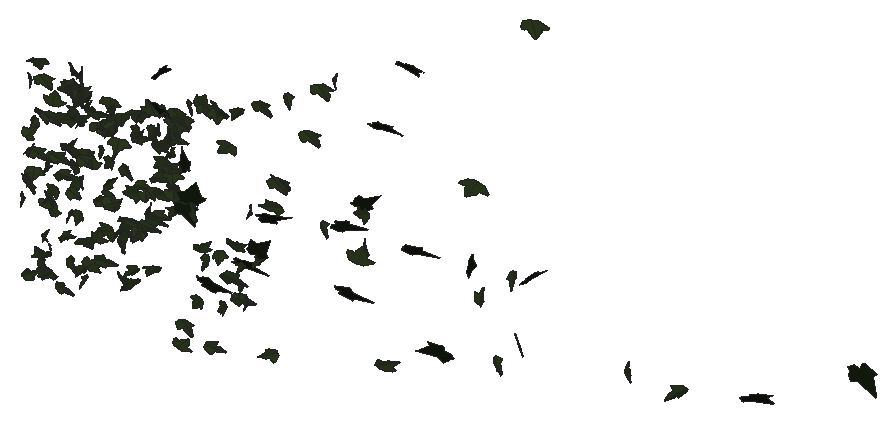
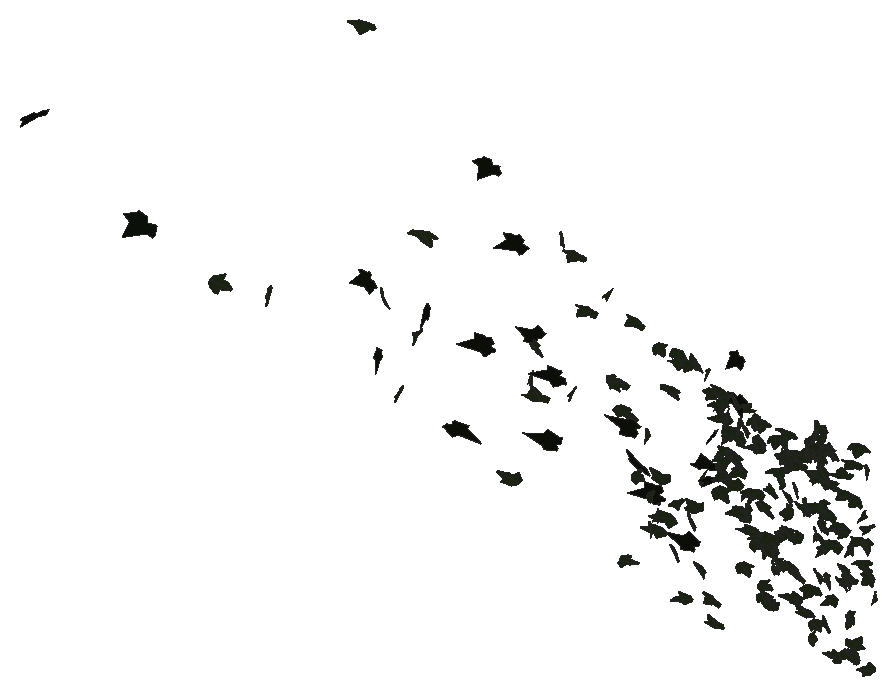
# SketchUp Ruby script. Lengths in millimetres.
U = 1.mm
M = Sketchup.active_model
def pt(a) = Geom::Point3d.new(a.map { |v| v * U })
def face(e, loops, mat)
  f = e.add_face(loops[0].map { |a| pt(a) })
  loops[1..].each { |l| e.add_face(l.map { |a| pt(a) }).erase! }
  f.material = f.back_material = mat if mat
  f
end
# faces: each face lists its corners as indices into pts; further lists are holes
def faces(e, pts, list, mat = nil) = list.each { |f| face(e, (f[0].is_a?(Array) ? f : [f]).map { |l| l.map { |i| pts[i] } }, mat) }
# xy, xz, yz: faces in a plane at the given z, y or x. An outline is a flat list of corners, or four numbers for a rectangle; further outlines are holes
def ring(l) = l.size == 4 ? [[l[0], l[1]], [l[2], l[1]], [l[2], l[3]], [l[0], l[3]]] : l.each_slice(2).to_a
def flat(e, list, mat, &to3) = list.each { |f| face(e, (f[0].is_a?(Array) ? f : [f]).map { |l| ring(l).map { |u, v| to3.(u, v) } }, mat) }
def xy(e, z, list, mat = nil) = flat(e, list, mat) { |x, y| [x, y, z] }
def xz(e, y, list, mat = nil) = flat(e, list, mat) { |x, z| [x, y, z] }
def yz(e, x, list, mat = nil) = flat(e, list, mat) { |y, z| [x, y, z] }
def lines(e, pts, list) = list.each { |a, b| e.add_line(pt(pts[a]), pt(pts[b])) }
# prism: a flat outline (further loops are holes) pulled along v
def prism(e, loops, v, mat = nil)
  f = face(e, loops, mat); d = Geom::Vector3d.new(v.map { |x| x * U })
  f.pushpull(f.normal.samedirection?(d) ? d.length : -d.length)
end
def box(e, o, s, mat = nil) = prism(e, [[o, [o[0] + s[0], o[1], o[2]], [o[0] + s[0], o[1] + s[1], o[2]], [o[0], o[1] + s[1], o[2]]]], [0, 0, s[2]], mat)
def at(x, y, z, deg = 0) = Geom::Transformation.translation(pt([x, y, z])) * Geom::Transformation.rotation(ORIGIN, Z_AXIS, deg.degrees)
def axes(o, x, y, z) = Geom::Transformation.new([*x, 0, *y, 0, *z, 0, *pt(o).to_a, 1])
def part(name) = M.definitions.add(name)
# library, detail: a bought-in or finely detailed component or shape, given as its bounding box
def library(name, o, s) = part(name).tap { |d| box(d.entities, o, s) }
def detail(e, o, s) = box(e.add_group.entities, o, s)
def put(e, d, t, mat = nil) = e.add_instance(d, t).tap { |i| i.material = mat if mat }
def group(e, t, mat = nil) = e.add_group.tap { |g| g.transformation = t; g.material = mat if mat }.entities
root = M.entities
M.materials.add("efeu1").color = [18, 25, 13]
M.materials.add("efeu2").color = [43, 57, 29]
c1 = part("ivyleaf_10")
p = [[0,12.8,-0.8],[-1.5,51.3,-10.9],[-4.9,51,-11.6],[-13.6,26.5,-7.3],[-13.2,15.9,-4.6],[-21.1,19.3,-7.2],
  [-29.5,16.3,-8.3],[-29.2,8.3,-6.2],[-19.7,-9.8,0.5],[-7.6,-13,4],[1,-12.2,5.8],[-0.4,51.1,-11.1],
  [-1.5,51.1,-10.9],[1,-12.4,5.9],[16.9,-12.4,3.5],[35.1,9.1,-5.1],[35,12.9,-6.1],[20.5,16.4,-4.9],
  [15.8,15,-3.8],[15.3,27.6,-7.1],[12.8,31.3,-7.8]]
faces(c1.entities,p,[[0,1,2,3,4,5,6,7,8,9,10],[11,12,0,13,14,15,16,17,18,19,20]],"efeu2")
c2 = part("ivyleaf_9")
p = [[39.1,54.8,31.7],[34.5,51.8,30.2],[-5.3,25.2,17.3],[-17.9,28.3,20.9],[-21.6,21.7,17],[-20.2,4.3,5.3],
  [-22.9,-0.3,2.5],[-17.1,-4,-0.6],[-2,-2.1,-1.2],[-0.7,-15.4,-10.1],[16.6,-22.3,-16.7],[21.1,-15.1,-12.5],
  [32.7,-10.7,-11],[46.1,-1.8,-6.6],[30.8,11.2,3.8]]
faces(c2.entities,p,[[0,1,2,3,4,5,6,7,8,9,10,11,12,13,14]],"efeu1")
put(root,c1,axes([1239.6,1052.6,288.6],[0.16019,-0.32764,-0.55839],[0.05337,0.5644,-0.32694],[1.23101,0.01817,0.08684]))
put(root,c1,axes([1265.3,1054.1,359.1],[0.11388,-0.04414,-0.63331],[-0.61555,0.54526,-0.06856],[1.03969,0.32766,0.02877]))
put(root,c1,axes([1251.3,1065.3,348],[-0.8892,0.39163,-0.24482],[0.3663,-0.15147,-0.6096],[-0.79905,-0.50525,-0.00702]))
put(root,c1,axes([1263.4,1066.4,467.4],[-0.03795,-0.71606,-0.12535],[0.02924,0.12496,-0.71624],[1.38322,-0.02229,0.0117]))
put(root,c1,axes([1252.7,1059.1,25.1],[-0.0891,-0.22264,0.63889],[0.20902,0.62942,0.22739],[-1.27057,0.11916,-0.0074]))
put(root,c1,axes([1256.2,1056.7,514.5],[0.46165,0.21093,-0.58955],[0.47216,0.54812,0.29818],[1.09414,-0.32553,0.12007]))
put(root,c1,axes([1273.6,1051.8,714.6],[0.36307,-0.38358,-0.48797],[-0.15599,0.49046,-0.41758],[1.17093,0.18427,0.09567]))
put(root,c1,axes([1269,1079.3,563],[0.15492,0.36895,-0.52964],[-0.1698,-0.52228,-0.37753],[-1.21667,0.11987,-0.01475]))
put(root,c1,axes([1275.1,1067.1,395.9],[0.8809,0.45478,-0.11108],[-0.15445,-0.0759,-0.64888],[-0.87748,0.46991,0.0027]))
put(root,c1,axes([1301.5,1079.7,102.7],[-0.83149,-0.33084,-0.35437],[-0.54732,-0.20719,0.54798],[-0.74282,0.523,-0.00709]))
put(root,c1,axes([1298.2,1060.5,785.8],[-1.01122,-0.36546,-0.08051],[0.13135,0.04172,-0.64486],[0.70001,-0.53577,0.0047]))
put(root,c1,axes([1280.6,1062.8,464.6],[0.59403,0.32673,0.47763],[0.61749,0.35055,-0.45183],[-0.91197,0.45018,0.00518]))
put(root,c1,axes([1300.4,1067.7,604.8],[-1.04499,0.31547,-0.19176],[0.30709,-0.10406,-0.63318],[-0.63197,-0.57221,0.00942]))
put(root,c1,axes([1297.4,1077.6,87.6],[0.62423,-0.2916,0.48272],[0.70851,-0.30752,-0.43871],[0.80626,0.49601,0.01179]))
put(root,c1,axes([1339.7,1065.9,59.1],[-0.8146,-0.17943,0.4451],[-0.7818,-0.17138,-0.46411],[0.47224,-0.59324,-0.00055]))
put(root,c1,axes([1306.1,1065.6,725.5],[0.86618,0.34796,0.36773],[0.54576,0.23032,-0.57285],[-0.79405,0.53787,0.00741]))
put(root,c1,axes([1325,1068.4,195.5],[0.1336,-0.59789,0.21849],[0.09631,-0.21388,-0.60152],[1.20767,0.0832,0.0238]))
put(root,c1,axes([1323.1,1068,63.3],[1.1405,-0.22119,-0.03341],[-0.05398,0.01964,-0.63871],[0.42231,0.59986,0.00859]))
put(root,c1,axes([1328,1060.2,425.4],[-0.0579,-0.29378,-0.60787],[0.16347,0.60186,-0.29517],[1.27448,-0.09054,0.01024]))
put(root,c1,axes([1335.3,1065,320],[-0.00784,-0.64851,-0.13381],[-0.01464,0.13385,-0.64847],[1.26016,-0.00248,-0.00837]))
put(root,c1,axes([1327.9,1068.9,160.2],[-0.63818,0.13904,0.55531],[0.74319,-0.41503,0.33971],[0.79666,0.49856,0.12793]))
put(root,c1,axes([1355.5,1053.2,316.1],[-0.27159,0.28396,-0.56339],[-0.60895,0.46526,0.31554],[1.03488,0.34829,0.03782]))
put(root,c1,axes([1333.9,1055.8,299.1],[0.71852,0.4355,-0.28324],[0.35775,0.21189,0.57636],[0.92173,-0.42173,-0.00291]))
put(root,c1,axes([1352.4,1069.9,352],[0.85257,-0.40554,-0.30883],[-0.43829,0.20578,-0.60426],[0.86549,0.50369,-0.00178]))
put(root,c1,axes([1332,1064.8,606.9],[0.80832,0.20292,0.45096],[0.74312,0.22718,-0.46996],[-0.57753,0.57632,0.02647]))
put(root,c1,axes([1357.4,1058.1,281],[1.04144,-0.3876,0.19874],[-0.29534,0.12469,0.67047],[-0.7746,-0.56867,0.01156]))
put(root,c1,axes([1356.4,1059.7,661.7],[1.04902,0.35634,-0.13418],[0.20507,0.08045,0.65628],[0.69505,-0.56155,0.00888]))
put(root,c1,axes([1349.1,1057.5,467.3],[0.3398,0.16685,-0.59298],[0.84375,0.39384,0.2443],[0.81397,-0.4779,-0.0057]))
put(root,c1,axes([1364.9,1055.4,480.9],[0.44094,0.27516,0.53506],[0.6765,0.40001,-0.35962],[-0.92391,0.42422,-0.00796]))
put(root,c1,axes([1411.9,1066.6,621],[0.66701,0.02989,-0.56874],[-1.08392,0.01961,-0.34992],[0.00198,0.66776,0.03573]))
put(root,c1,axes([1379.9,1066,418.4],[-0.48841,-0.15825,-0.61335],[1.04911,0.27023,-0.30036],[0.59392,-0.60748,0.02617]))
put(root,c1,axes([1374.9,1064.6,27.8],[0.19939,-0.05457,0.6283],[1.20027,0.00729,-0.10452],[0.00334,0.63693,0.05503]))
put(root,c1,axes([1415.5,1057.8,736.9],[0.50411,-0.35751,-0.46842],[-0.40172,0.42193,-0.44138],[1.04707,0.334,0.05618]))
put(root,c1,axes([1427.7,1059.4,733.6],[0.77838,-0.12558,-0.5347],[-0.95042,0.19254,-0.42719],[0.43522,0.64506,0.02342]))
put(root,c1,axes([1403.3,1052.5,218.6],[-0.32331,-0.2444,-0.60156],[0.58505,0.51743,-0.29703],[1.0885,-0.35071,-0.01903]))
put(root,c1,axes([1401.8,1069.3,518.8],[-0.97641,0.19167,-0.37538],[0.6599,-0.14427,-0.54755],[-0.45606,-0.61911,0.01138]))
put(root,c1,axes([1417.4,1066.8,292.8],[0.34392,-0.66787,0.01791],[0.00895,-0.01728,-0.69189],[1.27152,0.18077,0.00002]))
put(root,c1,axes([1416.8,1057.1,735.4],[-0.68286,0.52593,0.01901],[-0.02016,0.01579,-0.63666],[-1.0014,-0.35895,-0.00015]))
put(root,c1,axes([1416.9,1057.1,743],[-0.0608,-0.32113,-0.5712],[0.49185,0.51935,-0.30643],[1.14604,-0.23993,0.10121]))
put(root,c1,axes([1436.8,1060.3,799.3],[-0.86681,0.33583,0.4292],[-0.67636,0.24103,-0.56572],[-0.78632,-0.57754,0.01348]))
put(root,c1,axes([1429.1,1068.7,546.8],[-0.0112,-0.63791,0.03298],[0.00317,-0.033,-0.63793],[1.21569,-0.00579,0.00197]))
put(root,c1,axes([1444,1059.5,465.6],[0.24965,-0.12149,-0.63926],[-0.66353,0.53749,-0.17369],[1.04565,0.37008,0.04241]))
put(root,c1,axes([1439.1,1061.6,655.6],[0.79728,-0.3409,-0.40351],[-0.50996,0.30669,-0.53728],[0.86641,0.49422,0.05508]))
put(root,c1,axes([1414.1,1069.8,131],[0.54991,-0.24192,0.60536],[0.94435,-0.34786,-0.37585],[0.80472,0.57354,0.02739]))
put(root,c1,axes([1441.6,1064.2,700.2],[-1.03182,0.29658,0.16266],[-0.33597,0.01404,-0.61399],[-0.54914,-0.56585,0.07002]))
put(root,c1,axes([1429.4,1052,381.2],[0.19203,0.49755,0.43375],[0.19197,0.42201,-0.50755],[-1.2415,0.14221,-0.01139]))
put(root,c1,axes([1449.6,1060,418.3],[0.69375,-0.5007,-0.32821],[-0.37923,0.26089,-0.6193],[1.07446,0.41537,-0.00666]))
put(root,c1,axes([1449.6,1063.9,732.7],[-1.18296,-0.1435,0.01032],[-0.02191,0.004,-0.63788],[0.27294,-0.62163,-0.00649]))
put(root,c1,axes([1447.3,1057.2,757.7],[-0.83861,0.45851,0.01765],[-0.04594,0.00127,-0.6357],[-0.87207,-0.44098,0.01652]))
put(root,c1,axes([1444.6,1072.1,298.6],[0.93219,-0.42809,0.11067],[0.16016,-0.07188,-0.65051],[0.82615,0.49698,0.00124]))
put(root,c1,axes([1453.6,1064.8,709.4],[0.25157,-0.58425,-0.21694],[0.01868,0.22369,-0.59645],[1.18598,0.12041,0.05541]))
put(root,c1,axes([1440.5,1067.3,629],[-0.25397,-0.43712,0.49629],[0.55076,0.41665,0.44479],[-1.13178,0.30085,0.10509]))
put(root,c1,axes([1464.4,1070.6,119.1],[-0.29458,-0.51963,0.38028],[-0.07904,-0.38224,-0.53922],[1.22295,-0.14987,0.05675]))
put(root,c1,axes([1472.2,1051.3,420.4],[0.04343,-0.05324,0.7025],[-0.85764,0.53918,0.0555],[-1.03067,-0.45091,-0.01658]))
put(root,c1,axes([1461.3,1058.7,632.7],[-0.09736,-0.50073,-0.41595],[0.16387,0.40837,-0.50219],[1.22802,-0.09419,0.03403]))
put(root,c1,axes([1466.8,1056,771.8],[-0.50304,0.52876,0.26016],[-0.29957,0.21143,-0.58963],[-1.08081,-0.30471,0.04234]))
put(root,c1,axes([1464.7,1058,806.1],[0.14117,-0.5951,-0.25983],[0.07153,0.26502,-0.59624],[1.23377,0.05273,0.0643]))
put(root,c1,axes([1460.2,1084.6,75],[0.15411,-0.34471,0.5667],[0.30524,-0.54379,-0.35369],[1.22494,0.17887,0.01684]))
put(root,c1,axes([1455.1,1062.4,521.9],[-0.7574,-0.23527,-0.49108],[0.82287,0.23322,-0.46211],[0.62998,-0.58748,0.01321]))
put(root,c1,axes([1470.7,1062.7,714.4],[0.48976,-0.56848,-0.14836],[-0.00086,0.16178,-0.62067],[1.11816,0.24912,0.0645]))
put(root,c1,axes([1484.7,1052.8,745.3],[-0.07381,0.49339,0.40523],[-0.19245,0.3961,-0.49196],[-1.19979,-0.09389,0.05398]))
put(root,c1,axes([1474.8,1051.6,509.5],[0.40819,0.53764,0.39935],[0.27462,0.37239,-0.57883],[-1.2447,0.25848,0.00325]))
put(root,c1,axes([1483.2,1057.8,227.8],[-0.91923,-0.41566,-0.28145],[0.40242,0.18578,-0.63722],[0.86649,-0.52724,-0.00264]))
put(root,c1,axes([1490.9,1063.8,702.1],[-0.0473,-0.6374,-0.01661],[-0.00346,0.01669,-0.63788],[1.21351,-0.0248,-0.00246]))
put(root,c1,axes([1495.6,1060.7,732.5],[0.06628,-0.62539,-0.12878],[0.00532,0.12912,-0.62629],[1.21521,0.03354,0.00977]))
put(root,c1,axes([1494.1,1072.2,523.6],[0.57051,-0.49721,0.28868],[0.2419,-0.2602,-0.58014],[1.06716,0.3248,-0.02283]))
put(root,c1,axes([1506.7,1065.1,494.2],[1.02645,-0.14786,0.33847],[-0.62285,0.08644,0.55923],[-0.32593,-0.63085,-0.00271]))
put(root,c1,axes([1488.7,1065.2,140.1],[1.00816,-0.08575,-0.43916],[0.83742,-0.02382,0.53539],[-0.15472,-0.68767,0.03621]))
put(root,c1,axes([1500,1060.9,677.8],[-0.13491,-0.19303,0.65615],[1.15214,0.28929,0.1505],[-0.60579,0.59318,0.14012]))
put(root,c1,axes([1528.3,1058.7,247.3],[1.16473,-0.24836,0.05896],[-0.08475,0.04695,0.65992],[-0.47837,-0.61303,0.02665]))
put(root,c1,axes([1532.2,1052.7,381.8],[0.06111,-0.15718,0.61639],[0.04673,0.61702,0.15606],[-1.20976,0.01589,0.03717]))
put(root,c1,axes([1526.4,1058,641.1],[0.85884,0.33707,0.3113],[0.49371,0.17273,-0.56306],[-0.72028,0.5203,-0.01475]))
put(root,c1,axes([1545.7,1058,560.4],[0.43766,-0.53729,-0.27231],[-0.15774,0.26049,-0.58395],[1.1355,0.24327,0.02384]))
put(root,c1,axes([1564.7,1069.6,286.2],[0.82248,-0.30044,-0.52789],[-0.81753,0.30687,-0.52631],[0.8173,0.60931,0.00478]))
put(root,c1,axes([1532.8,1061.7,174.4],[0.00208,-0.01802,0.64676],[1.0337,0.3515,0.00888],[-0.66918,0.54291,0.01572]))
put(root,c1,axes([1557,1059.9,654],[-0.5159,-0.58819,-0.26203],[0.25601,0.22631,-0.64715],[1.19847,-0.30154,0.02544]))
put(root,c1,axes([1568.1,1068.9,408.1],[0.93797,-0.35342,-0.19578],[-0.30685,0.11112,-0.60645],[0.70506,0.51853,-0.00348]))
put(root,c1,axes([1568.5,1069,528.2],[0.80715,-0.45929,-0.17252],[-0.20746,0.13413,-0.62506],[0.91041,0.43776,0.01051]))
put(root,c1,axes([1564,1065,672.5],[-0.5616,-0.48275,-0.34445],[0.38498,0.27973,-0.56533],[1.06098,-0.35703,0.02281]))
put(root,c1,axes([1570.5,1060.7,638.8],[0.02134,-0.53491,-0.37796],[0.24625,0.37237,-0.52317],[1.22197,-0.0657,0.11203]))
put(root,c1,axes([1572.6,1048.8,452.4],[0.1687,-0.31802,0.67164],[-0.14685,0.6688,0.32686],[-1.40667,-0.10796,0.04643]))
put(root,c1,axes([1587.1,1055.9,706],[-0.62977,0.32557,0.43627],[-0.64225,0.27793,-0.46336],[-0.81294,-0.47179,0.0281]))
put(root,c1,axes([1570.1,1063.2,739.8],[1.19786,0.04433,0.095],[0.1826,-0.01054,-0.63072],[-0.08041,0.63644,-0.01706]))
put(root,c1,axes([1569.3,1059.6,650.4],[0.40078,0.25817,-0.65257],[0.76392,0.51456,0.3331],[1.09559,-0.45323,0.00646]))
put(root,c1,axes([1568.9,1050.9,387],[0.26831,0.07909,-0.65416],[0.78709,0.51018,0.15081],[0.97631,-0.43304,0.0582]))
put(root,c1,axes([1585,1061.4,725.1],[-0.09077,-0.61268,-0.18724],[0.16861,0.17965,-0.6104],[1.20757,-0.07114,0.07116]))
put(root,c1,axes([1590.5,1059.5,555.7],[0.3945,-0.47978,0.46203],[-0.30055,0.43469,0.52224],[-1.23154,-0.25977,0.02055]))
put(root,c1,axes([1592.5,1078.5,285.1],[0.25293,-0.54962,0.31428],[0.11792,-0.3083,-0.56535],[1.19918,0.14624,-0.01069]))
put(root,c1,axes([1590.7,1065.1,373.4],[0.23067,-0.47666,0.43195],[-0.14228,0.42614,0.49122],[-1.21597,-0.14029,0.02447]))
put(root,c1,axes([1601.1,1050.3,655.5],[0.11239,-0.33084,-0.56657],[-0.00846,0.56865,-0.33252],[1.24865,0.03363,0.04874]))
put(root,c1,axes([1597.5,1072.2,603.9],[0.97229,0.48886,-0.15534],[-0.21119,-0.10872,-0.70708],[-0.95312,0.52278,-0.00179]))
put(root,c1,axes([1630.1,1056.9,251.2],[0.11045,0.00502,0.65259],[-1.00304,0.38676,0.0439],[-0.73253,-0.52883,0.03829]))
put(root,c1,axes([1615.5,1057.2,308.5],[0.44434,-0.49596,0.3383],[-0.31731,0.29514,0.54774],[-1.09764,-0.28609,-0.02139]))
put(root,c1,axes([1617.7,1073.4,311.5],[0.33939,-0.6274,-0.0109],[-0.00691,0.0103,-0.65225],[1.19422,0.17836,-0.00067]))
put(root,c1,axes([1616.8,1063,703.6],[-0.69198,-0.52843,0.00032],[0.18451,-0.06709,-0.6305],[0.98863,-0.35734,0.1179]))
put(root,c1,axes([1631.6,1061.9,298.6],[0.69903,-0.45852,-0.26908],[-0.3442,0.19979,-0.5873],[0.95148,0.40914,-0.01477]))
put(root,c1,axes([1613,1076.1,126.6],[-0.78619,0.18815,0.45686],[0.80479,-0.17339,0.45375],[0.48639,0.59102,-0.01233]))
put(root,c1,axes([1633.8,1059.8,115.3],[-0.11644,-0.61834,0.14257],[0.02285,0.14208,0.62136],[-1.20749,0.06232,-0.00199]))
put(root,c1,axes([1618.6,1070.2,518.8],[0.45291,-0.1003,0.60244],[1.07049,-0.21592,-0.25813],[0.45287,0.61069,0.00767]))
put(root,c1,axes([1653.8,1062.3,303.1],[-0.85827,0.33204,-0.33354],[-0.51599,0.19432,0.56],[0.73216,0.52617,0.00367]))
put(root,c1,axes([1640.9,1060.1,353.4],[-1.12103,-0.04948,-0.26134],[0.49614,0.01864,-0.59109],[0.10047,-0.64413,0.00297]))
put(root,c1,axes([1669,1064,454.6],[0.7377,-0.23797,-0.54593],[-0.84337,0.31993,-0.45408],[0.75724,0.58815,0.02612]))
put(root,c1,axes([1654.9,1067.7,292.9],[0.52068,-0.48885,0.32679],[-0.30885,0.28366,0.56019],[-1.07565,-0.31808,-0.00266]))
put(root,c1,axes([1661.3,1071.2,183.3],[-0.15506,-0.36708,0.52453],[-0.14326,-0.51961,-0.37532],[1.21002,-0.10856,0.02278]))
put(root,c1,axes([1661.4,1069,145],[-0.50312,-0.5788,0.1034],[-0.07399,-0.09591,-0.6363],[1.11657,-0.26716,0.00443]))
put(root,c1,axes([1643.4,1057.8,339.9],[-0.49347,-0.05729,-0.58922],[1.11464,0.06902,-0.26443],[0.16437,-0.64004,0.02422]))
put(root,c1,axes([1676.9,1060.8,679.4],[0.69984,-0.53312,-0.12379],[-0.14146,0.09911,-0.64762],[1.03197,0.37512,-0.00482]))
put(root,c1,axes([1675.6,1063,736.3],[-0.76505,-0.4968,0.02458],[0.16377,-0.10059,-0.62568],[0.93239,-0.38997,0.13007]))
put(root,c1,axes([1692.7,1071.1,315.5],[-0.14066,-0.39629,0.5287],[-0.05978,-0.52928,-0.40112],[1.25608,-0.06957,0.04012]))
put(root,c1,axes([1674.9,1060.9,647.9],[0.05698,-0.04889,0.63892],[0.58809,0.56144,0.02849],[-1.06839,0.30643,0.04976]))
put(root,c1,axes([1682.8,1059.8,335.1],[0.50001,0.57552,0.13059],[0.10671,0.11796,-0.63264],[-1.11809,0.26863,-0.00198]))
put(root,c1,axes([1693.1,1064.4,672.1],[0.04109,-0.63533,0.02516],[0.04645,-0.02433,-0.63526],[1.20922,0.02252,0.02355]))
put(root,c1,axes([1695.3,1064.5,738.7],[-0.77176,-0.48926,0.03021],[0.08201,-0.07463,-0.63031],[0.92932,-0.39972,0.08071]))
put(root,c1,axes([1695.1,1063.1,745.9],[0.21901,-0.62928,0.02192],[0.00732,-0.02158,-0.63971],[1.19834,0.11514,-0.0001]))
put(root,c1,axes([1682.3,1060.1,489.1],[-0.39791,-0.19712,-0.57341],[0.84735,0.36184,-0.28673],[0.78339,-0.49151,0.01888]))
put(root,c1,axes([1710.7,1058.3,454],[0.21879,0.52621,-0.39602],[0.14483,0.3887,0.53858],[1.24502,-0.13769,0.00694]))
put(root,c1,axes([1698.2,1065.4,354.7],[-0.37633,-0.06266,-0.62741],[1.19756,0.02262,-0.20057],[0.07706,-0.65745,0.0529]))
put(root,c1,axes([1726.3,1061.4,425.8],[0.04743,-0.57452,-0.28179],[0.03211,0.28249,-0.57446],[1.21743,0.01493,0.02613]))
put(root,c1,axes([1725.5,1059,482.1],[0.03251,0.59871,0.28931],[-0.03018,0.28969,-0.59856],[-1.26517,0.00847,0.02171]))
put(root,c1,axes([1742.3,1067.1,218.5],[-0.55283,-0.52947,0.26685],[-0.23583,-0.23638,-0.6039],[1.10351,-0.31577,0.00463]))
put(root,c1,axes([1738.1,1063.1,761],[0.97832,0.35315,0.14437],[-0.27118,-0.047,0.62232],[0.67356,-0.53185,0.04086]))
put(root,c1,axes([1740,1062.5,701.3],[0.8401,-0.46826,-0.02029],[-0.00219,0.02678,-0.64328],[0.89202,0.44107,0.01752]))
put(root,c1,axes([1730.3,1060.7,388.2],[0.01617,-0.05379,0.66221],[1.21227,0.18898,0.00718],[-0.35957,0.63473,0.05398]))
put(root,c1,axes([1757.3,1061.4,710.6],[0.11878,-0.59673,-0.24058],[0.2022,0.24795,-0.58745],[1.20772,0.01718,0.12201]))
put(root,c2,axes([1772.2,1055.5,788.1],[0.83976,0.08611,-0.61161],[-1.15579,-0.07656,-0.4489],[-0.21432,0.75026,0.02439]))
put(root,c1,axes([1746.6,1063,407.4],[-0.42749,-0.15234,-0.61295],[0.96257,0.34629,-0.2714],[0.72001,-0.5534,-0.0011]))
put(root,c1,axes([1753.6,1059,541.7],[-0.46553,-0.28556,-0.55332],[0.74991,0.38932,-0.37511],[0.91759,-0.46305,0.02585]))
put(root,c1,axes([1742.1,1068.8,649.2],[-0.19896,-0.0025,0.74605],[1.36544,-0.20696,0.09984],[0.38945,0.72435,0.0311]))
put(root,c1,axes([1781.5,1070.2,594.5],[1.08344,-0.28984,-0.4175],[-0.6689,0.22834,-0.63774],[0.69872,0.66801,0.03685]))
put(root,c2,axes([1776.9,1043.5,920.1],[-0.23911,0.24535,-0.72939],[-0.57266,0.66455,0.27537],[1.34801,0.32583,-0.0124]))
put(root,c1,axes([1778.6,1061.5,784.9],[0.64533,-0.54519,-0.06077],[-0.00768,0.06896,-0.64119],[1.044,0.3375,0.03285]))
put(root,c1,axes([1784.2,1070.2,594.6],[1.10994,-0.47068,-0.14626],[-0.21959,0.08991,-0.74943],[0.91198,0.5945,-0.00245]))
put(root,c1,axes([1765.6,1061.1,483.7],[-0.3726,-0.21843,0.58171],[0.79239,0.40663,0.29281],[-0.87786,0.45975,0.0174]))
put(root,c1,axes([1789.8,1061.7,673.2],[-0.88409,-0.45378,-0.04907],[0.05486,0.04071,-0.64933],[0.86694,-0.46534,-0.00896]))
put(root,c1,axes([1805.6,1062.9,726],[0.01003,0.59662,-0.23108],[-0.02361,-0.23095,-0.59656],[-1.21745,0.0094,0.00966]))
put(root,c1,axes([1807.9,1068.6,567.4],[0.84778,0.50513,-0.06677],[-0.09144,-0.04665,-0.67347],[-0.96541,0.448,0.00516]))
put(root,c1,axes([1811.6,1055.9,648.1],[-0.20047,-0.50237,-0.46448],[0.20495,0.45192,-0.51321],[1.28593,-0.15035,0.00938]))
put(root,c1,axes([1811.9,1050.9,707.7],[0.2414,-0.4773,-0.50678],[0.17497,0.52209,-0.46871],[1.31333,0.01817,0.1556]))
put(root,c1,axes([1801.9,1060.8,592.7],[0.46909,0.26016,0.53209],[0.38521,0.50463,-0.34049],[-1.05938,0.29869,0.1118]))
put(root,c1,axes([1819.3,1061.9,756.3],[0.46689,0.56679,0.17941],[-0.11689,-0.16889,0.61752],[1.12542,-0.25268,-0.0103]))
put(root,c1,axes([1837.1,1057.1,522.8],[0.26708,-0.14811,-0.68645],[-0.87707,0.50878,-0.20399],[1.00846,0.48171,0.00439]))
put(root,c1,axes([1828.8,1073.2,451],[-0.53534,-0.61616,0.34771],[-0.28043,-0.31495,-0.67732],[1.31698,-0.31753,-0.00289]))
put(root,c1,axes([1817.7,1062.5,493.7],[0.80168,0.48824,-0.30348],[0.31387,0.25778,0.64363],[1.0481,-0.45065,0.03938]))
put(root,c1,axes([1824.5,1062.1,738.3],[-0.22184,0.61723,0.13735],[-0.02071,0.13768,-0.62797],[-1.20326,-0.11616,-0.01452]))
put(root,c1,axes([1811.9,1055.4,699.9],[-0.30875,-0.13455,-0.64567],[1.17413,0.20418,-0.19755],[0.4439,-0.63366,0.07344]))
put(root,c1,axes([1830.6,1061.5,741.2],[0.14979,0.61377,-0.17832],[-0.043,-0.17689,-0.61879],[-1.21567,0.08188,-0.00008]))
put(root,c1,axes([1834.2,1062.8,745.7],[0.89692,0.42567,-0.08953],[-0.22087,-0.00418,-0.63073],[-0.79785,0.47968,0.07396]))
put(root,c1,axes([1825,1059.6,792.1],[0.96009,0.05953,0.40313],[0.75111,0.08844,-0.50692],[-0.1932,0.63967,0.03257]))
put(root,c1,axes([1837.5,1069.7,-19.2],[1.09052,-0.06824,-0.29423],[0.55578,-0.03601,0.57704],[-0.14684,-0.64311,-0.00109]))
put(root,c2,axes([1867.5,1061.4,613.3],[-0.38231,-0.46113,0.58993],[0.44513,0.54159,0.50298],[-1.35376,0.3083,-0.00121]))
put(root,c1,axes([1855.9,1059.2,779.3],[-1.0216,-0.26976,-0.24742],[0.51137,0.00785,-0.59149],[0.4731,-0.591,0.10507]))
put(root,c1,axes([1850.2,1070.2,64],[0.97008,-0.03187,0.45632],[0.86676,-0.02867,-0.5107],[0.0816,0.68353,-0.00014]))
put(root,c2,axes([1862,1063,479.3],[-0.11303,-0.67875,-0.36334],[0.09717,0.36014,-0.68113],[1.46202,-0.07641,0.01718]))
put(root,c1,axes([1879.9,1058.2,837.7],[-0.39408,0.62099,-0.0177],[0.00903,-0.01707,-0.6546],[-1.1823,-0.20712,0.0009]))
put(root,c2,axes([1889.2,1060.2,507.9],[-1.03277,-0.20914,0.51751],[0.98453,0.08264,0.57584],[-0.39898,0.74529,0.08137]))
put(root,c1,axes([1908.5,1053,458],[-0.32519,0.64674,-0.35605],[-0.17701,0.3437,0.66893],[1.39389,0.19453,0.00188]))
put(root,c1,axes([1908.3,1071.7,163],[0.92561,-0.44559,-0.15978],[-0.21341,0.11412,-0.65956],[0.87528,0.49904,0.00816]))
put(root,c1,axes([1914.8,1066,846.4],[1.17398,-0.44004,-0.21224],[0.33176,-0.1211,0.75771],[-0.86861,-0.641,0.00255]))
put(root,c1,axes([1923.7,1062.2,350.9],[-0.631,-0.50986,0.30712],[0.30068,0.26356,0.60809],[-1.09218,0.36713,-0.01003]))
put(root,c1,axes([1939.8,1071.5,317.6],[0.83219,-0.63537,0.05467],[0.06753,-0.04195,-0.77128],[1.21183,0.43866,0.00544]))
put(root,c1,axes([1938.7,1061.2,847.4],[0.91726,0.33142,0.29887],[0.35426,0.25052,-0.57796],[-0.77196,0.50877,0.0899]))
put(root,c2,axes([1931.6,1074,228.8],[0.60823,-0.15421,0.67829],[1.11446,-0.34327,-0.35394],[0.71457,0.66662,-0.02534]))
put(root,c1,axes([1959.8,1060.5,26.7],[0.2508,0.19349,0.62545],[0.69275,0.50866,-0.23405],[-1.0357,0.38708,-0.00509]))
put(root,c1,axes([1997.4,1057.7,863.6],[-1.18502,0.36924,0.3488],[-0.58393,0.16635,-0.7238],[-0.77042,-0.69403,0.01209]))
put(root,c1,axes([1979.3,1066,843.1],[0.95014,0.42513,0.07231],[0.09992,0.04988,-0.65571],[-0.81462,0.50197,0.00391]))
put(root,c1,axes([1990.2,1067.6,355.7],[0.46195,0.60528,-0.1459],[-0.12869,-0.13004,-0.65198],[-1.17795,0.25158,0.01401]))
put(root,c1,axes([2015.4,1060.4,181.9],[0.57149,-0.55214,-0.34084],[-0.31226,0.29875,-0.62851],[1.1948,0.34218,-0.00123]))
put(root,c1,axes([2024.6,1071.2,739.6],[1.14256,-0.09688,-0.30791],[-0.58164,0.03868,-0.60803],[0.19774,0.67358,-0.00937]))
put(root,c1,axes([2021.2,1071.1,287.6],[-0.58569,0.05623,-0.71935],[1.36573,-0.05784,-0.31151],[-0.14345,-0.78027,-0.02874]))
put(root,c1,axes([2060,1078.7,870.1],[-0.32093,-0.55856,0.33637],[-0.05809,-0.34029,-0.58037],[1.23957,-0.16056,0.05989]))
put(root,c1,axes([2052,1063.3,406.3],[-0.87849,-0.16084,0.47091],[0.88267,0.09378,0.48663],[-0.3433,0.65271,0.04612]))
put(root,c1,axes([2085.1,1076,348.7],[-0.21661,-0.59526,0.33256],[-0.08872,-0.32958,-0.60588],[1.29468,-0.12218,0.01412]))
put(root,c1,axes([2087.1,1046.6,271],[0.058,-0.14897,-0.70715],[0.03597,0.7077,-0.14827],[1.37491,-0.01223,0.03371]))
put(root,c1,axes([2060.6,1066.2,227.7],[-0.19267,-0.04001,-0.67305],[1.28173,0.02672,-0.10288],[0.06168,-0.6801,0.03555]))
put(root,c1,axes([2103.2,1060.2,230.3],[0.20647,-0.37254,-0.59541],[-0.2301,0.58357,-0.38716],[1.31676,0.16039,0.0257]))
put(root,c2,axes([2068.1,1066.4,353.2],[1.2626,-0.03506,0.43888],[0.83232,-0.03928,-0.6642],[0.09687,0.79447,-0.01347]))
put(root,c1,axes([2114,1062.7,551.2],[0.15182,-0.54033,-0.43857],[0.07274,0.44417,-0.54029],[1.32247,0.0376,0.08006]))
put(root,c1,axes([2149.8,1074.1,391],[-0.04186,-0.40986,0.57044],[0.06508,-0.57067,-0.4087],[1.33525,0.01496,0.0378]))
put(root,c2,axes([2141.4,1059.9,414.4],[-0.65749,0.50343,0.53288],[0.57146,-0.44023,0.61056],[1.27279,0.45771,0.00114]))
put(root,c1,axes([2141.9,1071.6,923.8],[0.87066,-0.00612,0.51026],[0.96004,0.10904,-0.45094],[-0.14685,0.67658,0.07729]))
put(root,c1,axes([2198.9,1072,80.3],[0.31192,0.15728,-0.66961],[-0.89486,-0.4768,-0.22707],[-0.95548,0.49789,-0.00593]))
put(root,c1,axes([2213.7,1067.9,595.5],[0.6158,0.04676,-0.639],[-1.21447,0.08778,-0.31669],[0.10946,0.71085,0.08114]))
put(root,c2,axes([2167.2,1062.3,544.4],[0.89715,0.48791,-0.37327],[0.40501,0.31167,0.67615],[1.09678,-0.5142,0.05565]))
put(root,c1,axes([2250.6,1063.8,678.6],[-0.54363,0.17518,-0.63915],[-1.08241,0.29249,0.33434],[0.64748,0.63604,0.02229]))
put(root,c1,axes([2214,1061.7,685.8],[0.99157,0.25514,0.41856],[0.68529,0.21528,-0.57942],[-0.63303,0.63268,0.02837]))
put(root,c1,axes([2252.1,1069.6,990.1],[-0.00796,0.69932,-0.06517],[0.00451,-0.06516,-0.69933],[-1.3367,-0.00438,-0.00197]))
put(root,c1,axes([2335.6,1062.1,892],[0.95819,0.22872,0.47666],[0.77357,0.25347,-0.55094],[-0.64347,0.64531,0.04746]))
put(root,c1,axes([2381.6,1063.3,1069.7],[1.0723,0.284,0.34909],[0.5894,0.16115,-0.63093],[-0.62141,0.64291,0.00394]))
put(root,c1,axes([2396.6,1063.8,596.6],[-0.21532,0.72862,0.06154],[-0.0412,0.05891,-0.73725],[-1.39104,-0.11453,0.01231]))
put(root,c1,axes([2446.6,1060.1,1110],[-0.08766,0.19606,0.70271],[-0.91792,0.52011,-0.17672],[-1.04178,-0.47477,0.09658]))
put(root,c2,axes([2459.1,1060.6,623.6],[0.30575,0.36443,-0.67271],[0.50226,0.6188,0.39825],[1.36674,-0.30893,0.00414]))
put(root,c2,axes([2469.1,1069.1,390.2],[0.84275,-0.17669,0.66191],[1.19866,-0.20514,-0.4761],[0.51307,0.76949,0.02506]))
put(root,c1,axes([2528.7,1067.8,523.4],[1.45132,0.24788,-0.21122],[0.38296,0.06424,0.80184],[0.48734,-0.78867,-0.00107]))
put(root,c1,axes([2563.5,1056.9,700.4],[0.64213,-0.35819,-0.59038],[-0.7725,0.42872,-0.49207],[1.06324,0.52781,-0.00096]))
put(root,c1,axes([2567.3,1054.5,582.7],[-0.34859,0.23512,0.70547],[-0.78497,0.57244,-0.29787],[-1.17762,-0.45117,-0.01028]))
put(root,c2,axes([2548.9,1054.6,724.8],[-0.0905,-0.04459,0.76434],[1.32749,0.31328,0.06167],[-0.6009,0.6988,0.02112]))
put(root,c2,axes([2611,1054.3,1025.4],[1.31367,0.12291,0.31894],[0.58889,0.08065,-0.70073],[-0.27637,0.75608,0.02289]))
put(root,c1,axes([2632.9,1055.4,196.4],[-0.59974,-0.40181,0.57351],[0.6732,0.45143,0.51064],[-1.1502,0.47373,-0.00017]))
put(root,c2,axes([2716.2,1064.2,1265.4],[1.37231,0.23572,-0.12573],[-0.249,-0.00395,-0.75773],[-0.4433,0.73192,0.0364]))
put(root,c2,axes([2729.9,1060.8,633.2],[1.17674,0.06117,0.53264],[0.99764,0.10175,-0.62017],[-0.21426,0.80972,0.03769]))
put(root,c2,axes([2851.3,1072.5,317.8],[-0.07453,0.10134,-0.79983],[-1.13316,-0.54355,-0.03972],[-1.03457,0.58805,0.10112]))
put(root,c2,axes([2973.6,1050.4,670.5],[0.20147,0.00489,-0.89003],[-1.18493,0.64092,-0.07053],[1.21051,0.62656,0.07909]))
put(root,c1,axes([2978.7,1071,940],[1.54449,0.15388,-0.26291],[-0.49345,-0.04384,-0.82597],[-0.30436,0.85192,0.00499]))
put(root,c1,axes([3014.5,1046.9,560.7],[0.06891,0.51412,-0.64767],[0.15491,0.64293,0.5149],[1.56616,-0.08622,-0.02243]))
put(root,c1,axes([3066.1,1064.6,360.9],[-0.29721,0.81876,0.06978],[-0.02452,0.06859,-0.83352],[-1.56371,-0.1567,-0.0002]))
put(root,c1,axes([3118.4,1080.3,672.5],[0.8993,-0.57439,0.48351],[0.57201,-0.37881,-0.74374],[1.30943,0.55996,-0.00717]))
put(root,c2,axes([3151.7,1061.6,459.9],[0.72379,-0.18969,-0.73007],[-1.23107,0.3386,-0.42492],[0.73853,0.75032,0.00718]))
put(root,c2,axes([3195.9,1054,697.4],[-0.25484,0.58279,-0.65196],[-0.36803,0.6235,0.59706],[1.62309,0.23288,0.03302]))
put(root,c1,axes([3206.6,1062.2,1581.4],[1.30139,0.45294,0.15613],[0.23119,0.09929,-0.82005],[-0.88203,0.69432,0.01542]))
put(root,c1,axes([3589.4,1044.9,515.2],[-0.43195,0.46707,0.73714],[-0.70633,0.63769,-0.51832],[-1.50315,-0.43387,0.03174]))
put(root,c1,axes([3767.9,1083.7,499.2],[-0.18045,-0.54965,0.7909],[-0.27932,-0.77719,-0.55773],[1.81164,-0.17458,-0.00721]))
put(root,c2,axes([4058.2,1055.6,590.1],[1.30411,0.61936,0.36595],[0.50185,0.25399,-0.92359],[-1.27387,0.73413,0.01079]))
put(root,c2,axes([4474.5,1066,826.4],[0.21069,-0.93705,-0.4706],[-0.10445,0.46739,-0.94357],[1.99293,0.12356,0.0003]))
